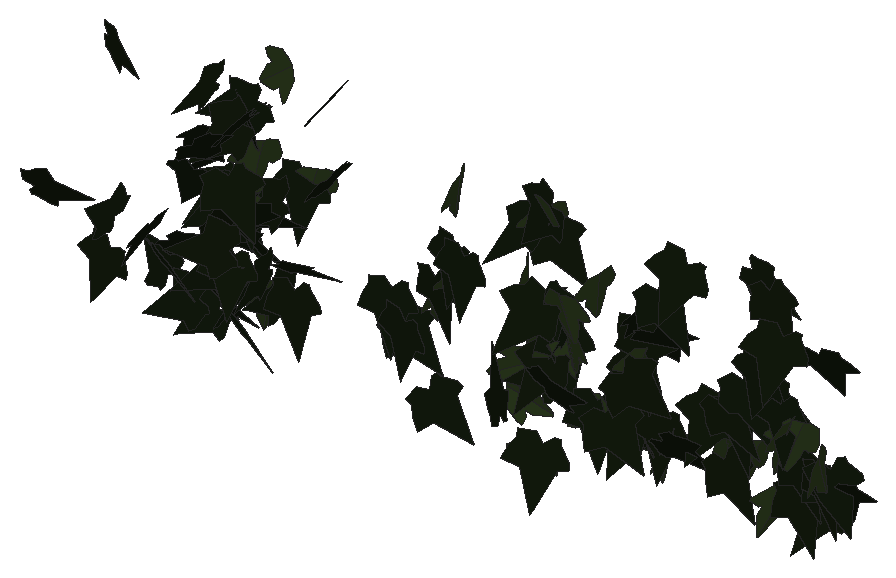
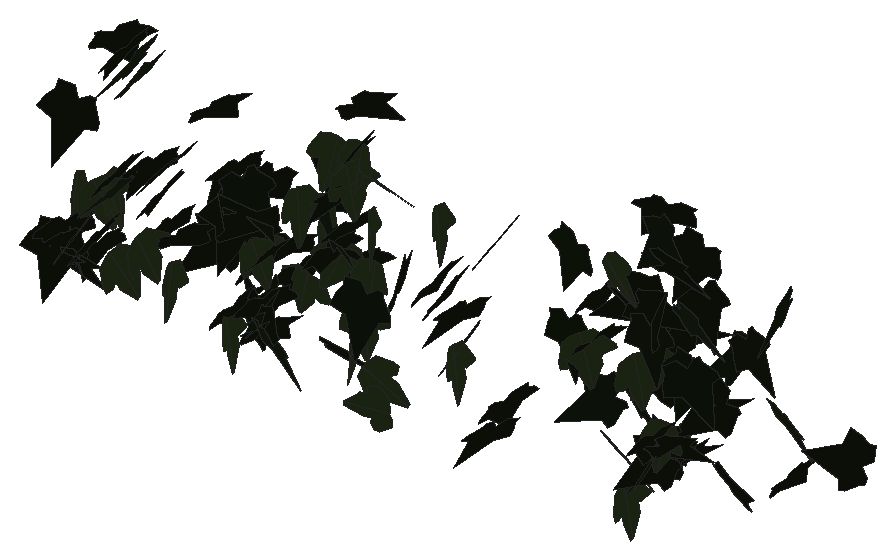
# SketchUp Ruby script. Lengths in inches.
U = 1.inch
M = Sketchup.active_model
def pt(a) = Geom::Point3d.new(a.map { |v| v * U })
def face(e, loops, mat)
  f = e.add_face(loops[0].map { |a| pt(a) })
  loops[1..].each { |l| e.add_face(l.map { |a| pt(a) }).erase! }
  f.material = f.back_material = mat if mat
  f
end
# faces: each face lists its corners as indices into pts; further lists are holes
def faces(e, pts, list, mat = nil) = list.each { |f| face(e, (f[0].is_a?(Array) ? f : [f]).map { |l| l.map { |i| pts[i] } }, mat) }
# xy, xz, yz: faces in a plane at the given z, y or x. An outline is a flat list of corners, or four numbers for a rectangle; further outlines are holes
def ring(l) = l.size == 4 ? [[l[0], l[1]], [l[2], l[1]], [l[2], l[3]], [l[0], l[3]]] : l.each_slice(2).to_a
def flat(e, list, mat, &to3) = list.each { |f| face(e, (f[0].is_a?(Array) ? f : [f]).map { |l| ring(l).map { |u, v| to3.(u, v) } }, mat) }
def xy(e, z, list, mat = nil) = flat(e, list, mat) { |x, y| [x, y, z] }
def xz(e, y, list, mat = nil) = flat(e, list, mat) { |x, z| [x, y, z] }
def yz(e, x, list, mat = nil) = flat(e, list, mat) { |y, z| [x, y, z] }
def lines(e, pts, list) = list.each { |a, b| e.add_line(pt(pts[a]), pt(pts[b])) }
# prism: a flat outline (further loops are holes) pulled along v
def prism(e, loops, v, mat = nil)
  f = face(e, loops, mat); d = Geom::Vector3d.new(v.map { |x| x * U })
  f.pushpull(f.normal.samedirection?(d) ? d.length : -d.length)
end
def box(e, o, s, mat = nil) = prism(e, [[o, [o[0] + s[0], o[1], o[2]], [o[0] + s[0], o[1] + s[1], o[2]], [o[0], o[1] + s[1], o[2]]]], [0, 0, s[2]], mat)
def at(x, y, z, deg = 0) = Geom::Transformation.translation(pt([x, y, z])) * Geom::Transformation.rotation(ORIGIN, Z_AXIS, deg.degrees)
def axes(o, x, y, z) = Geom::Transformation.new([*x, 0, *y, 0, *z, 0, *pt(o).to_a, 1])
def part(name) = M.definitions.add(name)
# library, detail: a bought-in or finely detailed component or shape, given as its bounding box
def library(name, o, s) = part(name).tap { |d| box(d.entities, o, s) }
def detail(e, o, s) = box(e.add_group.entities, o, s)
def put(e, d, t, mat = nil) = e.add_instance(d, t).tap { |i| i.material = mat if mat }
def group(e, t, mat = nil) = e.add_group.tap { |g| g.transformation = t; g.material = mat if mat }.entities
root = M.entities
M.materials.add("efeu1").color = [18, 25, 13]
M.materials.add("efeu2").color = [43, 57, 29]
c1 = part("ivyleaf_9")
p = [[1.54,2.16,1.25],[1.36,2.04,1.19],[-0.21,0.99,0.68],[-0.71,1.11,0.82],[-0.85,0.86,0.67],[-0.8,0.17,0.21],
  [-0.9,-0.01,0.1],[-0.67,-0.16,-0.02],[-0.08,-0.08,-0.05],[-0.03,-0.6,-0.4],[0.65,-0.88,-0.66],[0.83,-0.6,-0.49],
  [1.29,-0.42,-0.43],[1.8125,-0.07,-0.26],[1.21,0.44,0.15]]
faces(c1.entities,p,[[0,1,2,3,4,5,6,7,8,9,10,11,12,13,14]],"efeu1")
c2 = part("ivyleaf_10")
p = [[0,0.5,-0.03],[-0.0625,2.02,-0.43],[-0.19,2.01,-0.46],[-0.54,1.05,-0.29],[-0.52,0.625,-0.18],[-0.83,0.76,-0.28],
  [-1.16,0.64,-0.33],[-1.15,0.33,-0.24],[-0.77,-0.39,0.02],[-0.3,-0.51,0.16],[0.04,-0.48,0.23],[-0.02,2.01,-0.4375],
  [-0.06,2.01,-0.43],[0.04,-0.49,0.23],[0.67,-0.49,0.14],[1.38,0.36,-0.2],[1.375,0.51,-0.24],[0.81,0.65,-0.19],
  [0.62,0.59,-0.15],[0.6,1.09,-0.28],[0.5,1.23,-0.31]]
faces(c2.entities,p,[[0,1,2,3,4,5,6,7,8,9,10],[11,12,0,13,14,15,16,17,18,19,20]],"efeu2")
put(root,c1,axes([1.47,220.37,250.14],[0.26717,-0.08077,0.36252],[0.37184,-0.06164,-0.26897],[0.10521,0.42297,0.03003]))
put(root,c1,axes([2.86,221.11,253.88],[0.33845,-0.15034,-0.27202],[-0.23301,0.15192,-0.35966],[0.22774,0.37887,0.03628]))
put(root,c1,axes([3.35,220.45,249.21],[-0.09676,-0.39725,0.15906],[-0.03153,-0.15019,-0.42349],[0.45865,-0.09413,0.00444]))
put(root,c1,axes([3.79,220.04,250.37],[-0.22269,0.31879,0.22081],[-0.16184,0.15477,-0.39303],[-0.38069,-0.25228,0.03791]))
put(root,c1,axes([4.49,220.96,248.875],[-0.05804,0.18798,0.40413],[-0.27352,0.30338,-0.18905],[-0.37753,-0.24869,0.07484]))
put(root,c1,axes([4.79,222,251.98],[-0.02197,0.39044,-0.19833],[-0.12796,-0.18866,-0.38857],[-0.4515,0.03446,0.11977]))
put(root,c1,axes([5.03,221.85,253.23],[-0.38794,0.2394,-0.05584],[0.00925,-0.08289,-0.44402],[-0.26482,-0.35361,0.06628]))
put(root,c1,axes([5.04,222.57,250.34],[-0.38442,-0.18908,0.17018],[-0.14265,-0.09954,-0.41843],[0.22931,-0.3789,0.025]))
put(root,c1,axes([5.12,221.42,251.63],[0.10444,0.39445,0.16206],[0.00715,0.15841,-0.42128],[-0.45799,0.09242,0.03038]))
put(root,c2,axes([5.23,222.28,250.46],[-0.46353,0.07045,-0.00756],[0.00451,-0.01941,-0.45193],[-0.07636,-0.42882,0.01921]))
put(root,c1,axes([5.52,219.09,251.15],[-0.20155,0.34672,-0.19227],[0.07162,-0.17394,-0.40888],[-0.41828,-0.19686,0.02264]))
put(root,c1,axes([5.3,222.53,250.45],[-0.00279,-0.422,-0.10976],[-0.0063,0.10556,-0.43884],[0.46975,-0.00109,-0.00654]))
put(root,c1,axes([5.28,220.2,250.21],[0.40085,0.17066,0.15545],[0.13196,0.0911,-0.42372],[-0.20644,0.38962,0.03099]))
put(root,c1,axes([5.38,222.49,249.8],[0.27941,-0.33969,-0.08639],[-0.06872,0.05588,-0.44374],[0.37137,0.26592,-0.01711]))
put(root,c1,axes([5.41,222,249.67],[0.44642,0.07487,0.11749],[0.1211,0.01475,-0.43684],[-0.08221,0.42826,-0.00549]))
put(root,c1,axes([5.9,221.89,252.59],[-0.04503,0.43281,-0.01328],[0.00329,-0.01253,-0.4522],[-0.46763,-0.04176,-0.00191]))
put(root,c1,axes([6.08,221.93,253.1],[-0.07388,-0.04884,-0.44387],[-0.27919,-0.34049,0.08362],[-0.37055,0.26628,0.0255]))
put(root,c1,axes([5.97,221.91,252.3],[0.17673,-0.27189,0.30943],[-0.11011,0.28275,0.32704],[-0.42113,-0.18803,0.04434]))
put(root,c2,axes([6,222.24,251.78],[-0.21211,-0.44557,0.08049],[0.00836,-0.09273,-0.49126],[0.4527,-0.20706,0.04679]))
put(root,c1,axes([6.29,221.07,251.24],[-0.48318,0.06047,0.1135],[-0.11269,0.01356,-0.48695],[-0.06197,-0.49614,0.00052]))
put(root,c1,axes([6.19,219.76,252.41],[0.24309,0.17741,-0.34034],[-0.30731,-0.16455,-0.29632],[-0.25919,0.36149,0.03214]))
put(root,c1,axes([5.76,219.03,250.67],[0.36836,-0.2572,0.08541],[0.07301,-0.04674,-0.44425],[0.2823,0.34769,0.00346]))
put(root,c1,axes([6.16,220.58,248.72],[-0.23896,-0.23043,0.30706],[-0.12442,-0.28442,-0.32065],[0.38487,-0.23502,0.08698]))
put(root,c1,axes([6.3,219.71,249.39],[-0.21293,-0.16359,0.36562],[-0.2606,-0.25696,-0.26509],[0.32781,-0.31054,0.02675]))
put(root,c2,axes([6.29,222.2,248.55],[0.00629,-0.49925,0.02656],[0.03614,-0.02604,-0.49801],[0.49865,0.00819,0.03576]))
put(root,c2,axes([6.24,221.17,251.37],[-0.29768,-0.30364,-0.26303],[0.20864,0.16291,-0.42418],[0.3433,-0.3623,0.02972]))
put(root,c1,axes([5.99,220.79,248.86],[0.24443,-0.2247,0.30766],[0.27772,-0.15523,-0.32723],[0.28955,0.33858,0.05415]))
put(root,c2,axes([6.64,222.22,253.96],[0.28525,-0.16574,-0.37572],[-0.32389,0.19042,-0.3299],[0.25245,0.43159,0.00127]))
put(root,c1,axes([6.42,219.5,253.23],[0.25967,0.35435,0.07952],[0.03807,0.06847,-0.44525],[-0.38966,0.24284,0.0095]))
put(root,c1,axes([6.69,220.3,248.96],[-0.0441,0.36683,0.2394],[-0.07348,0.22291,-0.38199],[-0.46192,-0.07048,0.03791]))
put(root,c1,axes([6.78,220.55,253.38],[-0.49533,-0.01361,0.0668],[-0.06663,-0.007,-0.49549],[0.01442,-0.49977,0.00512]))
put(root,c1,axes([6.49,220.02,250.96],[0.10918,0.00626,0.43997],[0.30484,0.32301,-0.07512],[-0.34039,0.29129,0.07384]))
put(root,c1,axes([6.91,220.03,250.25],[-0.06009,-0.06788,-0.4431],[-0.06801,-0.4237,0.07876],[-0.46095,0.07136,0.04615]))
put(root,c1,axes([7.1875,219.61,250.93],[-0.26721,-0.05434,0.36778],[-0.36126,-0.11745,-0.26216],[0.13713,-0.4153,0.02602]))
put(root,c1,axes([6.92,219.92,253.49],[0.17163,0.26338,0.31988],[0.06673,0.31077,-0.30996],[-0.43221,0.15257,0.07916]))
put(root,c1,axes([6.91,220.12,250.38],[-0.13899,-0.40978,-0.07161],[0.02156,0.0659,-0.4467],[0.44825,-0.13023,-0.00072]))
put(root,c1,axes([6.71,220.5,248.67],[0.37999,-0.25111,0.05068],[0.04163,-0.02988,-0.44955],[0.27311,0.35394,-0.002]))
put(root,c1,axes([7.32,221.39,249.08],[-0.3702,0.24263,0.11794],[-0.11124,0.05059,-0.43637],[-0.267,-0.35748,0.01829]))
put(root,c1,axes([7.39,220.69,250.02],[-0.39715,0.19524,-0.13105],[0.12013,-0.05921,-0.433],[-0.22034,-0.38419,0.00014]))
put(root,c2,axes([7.56,222.13,251.7],[-0.31625,-0.36613,0.12622],[-0.04899,-0.12383,-0.48194],[0.38417,-0.3172,0.04245]))
put(root,c1,axes([7.43,221.9375,251.73],[-0.06077,-0.49604,0.01598],[-0.00384,-0.01563,-0.49974],[0.49628,-0.06086,-0.00191]))
put(root,c1,axes([8,220.39,252.03],[-0.43539,0.15483,0.05436],[-0.0519,0.02068,-0.44912],[-0.16869,-0.40599,-0.00215]))
put(root,c1,axes([7.53,221.13,250.01],[0.44332,0.04848,0.14098],[0.12072,0.15081,-0.40811],[-0.09799,0.40513,0.13505]))
put(root,c1,axes([7.5,219.85,251.78],[0.36684,0.06871,0.27344],[0.27106,0.08206,-0.35951],[-0.11254,0.42163,0.02541]))
put(root,c1,axes([8.09,221.88,251.94],[-0.05812,0.43159,0.00808],[-0.00084,0.00773,-0.45233],[-0.46619,-0.05382,-0.00019]))
put(root,c1,axes([8.06,221.7,253.73],[0.04337,0.36601,0.24088],[-0.01546,0.23361,-0.38134],[-0.46754,0.02622,0.03496]))
put(root,c1,axes([8.03,218.65,253.36],[-0.11834,-0.332,-0.35464],[0.26166,0.26397,-0.33444],[0.4093,-0.26475,0.11127]))
put(root,c1,axes([9.52,218.99,250.98],[0.02229,-0.49911,-0.01969],[-0.00044,0.01969,-0.49961],[0.4995,0.02229,0.00044]))
put(root,c1,axes([9.57,222.18,249.65],[-0.02982,-0.49833,-0.02789],[-0.00275,0.0281,-0.4992],[0.4991,-0.02962,-0.00442]))
put(root,c1,axes([9.79,222.29,248.98],[0.14741,-0.36704,-0.30586],[0.02144,0.32485,-0.37949],[0.47729,0.09876,0.11151]))
put(root,c2,axes([10.91,222.18,250.25],[0.08245,-0.48558,-0.08612],[-0.00039,0.08725,-0.49233],[0.49315,0.08125,0.01401]))
put(root,c1,axes([10.87,222.05,250.44],[0.1796,-0.45991,0.07895],[0.01719,-0.07801,-0.49358],[0.46632,0.18,-0.01221]))
put(root,c2,axes([11.66,221.8,253.18],[0.13435,-0.46763,-0.1152],[-0.00065,0.11942,-0.48553],[0.48161,0.13061,0.03148]))
put(root,c1,axes([11.49,221.93,251.4],[0.02545,-0.45539,0.20488],[0.00017,-0.20514,-0.45598],[0.49935,0.02328,-0.01029]))
put(root,c1,axes([11.93,221.66,251.47],[0.02249,-0.48468,0.12075],[0.0066,-0.12058,-0.4852],[0.49945,0.02342,0.00097]))
put(root,c1,axes([12.3,219.2,251.12],[0.03829,-0.45461,0.2046],[0.03718,-0.20202,-0.45586],[0.49714,0.05012,0.01833]))
put(root,c2,axes([13.09,222.22,249.09],[0.25296,0.01557,-0.43101],[-0.4263,0.08479,-0.24713],[0.06539,0.49251,0.05617]))
put(root,c1,axes([12.85,219.42,249.57],[0.17281,-0.34389,-0.31917],[0.00105,0.34042,-0.36622],[0.46919,0.12591,0.11838]))
put(root,c2,axes([12.85,222.25,248.3125],[0.05932,0.01609,0.49621],[0.48469,0.10636,-0.06139],[-0.10753,0.48829,-0.00298]))
put(root,c1,axes([13.43,222.05,250.76],[0.09261,0.48926,0.04529],[0.00191,0.04572,-0.4979],[-0.49135,0.09239,0.0066]))
put(root,c2,axes([13.73,222.05,249.7],[0.16228,-0.415,-0.2268],[0.0164,0.24458,-0.43579],[0.47265,0.134,0.09299]))
put(root,c2,axes([13.8125,221.4,250.93],[-0.47961,0.12763,0.06072],[-0.05992,0.01094,-0.49628],[-0.12801,-0.48331,0.0048]))
put(root,c1,axes([14.19,222.18,249.31],[-0.41889,0.17262,0.2115],[-0.23301,-0.02421,-0.44173],[-0.14226,-0.46863,0.10072]))
put(root,c1,axes([14.05,221.41,253.29],[-0.4968,0.02688,-0.04966],[0.04135,-0.1263,-0.48202],[-0.03846,-0.48304,0.12327]))
put(root,c2,axes([13.9,221.28,252.04],[0.21851,-0.43788,-0.10254],[0.03939,0.1322,-0.48059],[0.448,0.20195,0.09227]))
put(root,c2,axes([14.12,221.46,253.7],[-0.46501,0.17551,0.05444],[-0.04867,0.0252,-0.49699],[-0.17719,-0.46751,-0.00635]))
put(root,c2,axes([14.13,221.77,253.32],[-0.16561,-0.46911,0.05011],[-0.00657,-0.05081,-0.49737],[0.47173,-0.16539,0.01066]))
put(root,c1,axes([14.43,219.74,249.53],[-0.02796,-0.30077,0.39844],[0.04414,0.39601,0.30204],[-0.49726,0.05207,0.00441]))
put(root,c1,axes([14.27,221.68,253.53],[-0.10974,-0.32767,0.36137],[-0.0383,-0.36347,-0.3412],[0.4863,-0.10257,0.05468]))
put(root,c1,axes([14.24,221.77,252.95],[0.13061,-0.40859,-0.2569],[0.05637,0.27723,-0.41227],[0.47934,0.07873,0.11848]))
put(root,c1,axes([14.56,221.15,251.74],[0.11651,-0.45436,-0.17315],[0.02718,0.18386,-0.46417],[0.48548,0.09875,0.06754]))
put(root,c1,axes([15.07,220.71,250.62],[-0.4748,-0.12796,-0.09052],[0.09484,-0.00461,-0.4909],[0.1248,-0.48333,0.02865]))
put(root,c2,axes([15.27,219.84,248.75],[-0.48283,-0.05888,0.11581],[-0.11103,-0.04437,-0.48549],[0.06745,-0.49453,0.02977]))
put(root,c1,axes([15.32,221.02,251.52],[-0.3913,0.24091,-0.1971],[0.17319,-0.09457,-0.45941],[-0.25863,-0.42781,-0.00944]))
put(root,c2,axes([15.09,220.76,250.7],[-0.44054,-0.14074,-0.19004],[0.2038,-0.02211,-0.45605],[0.11996,-0.47927,0.07685]))
put(root,c1,axes([15.04,221.23,251.01],[-0.00964,-0.49252,-0.0856],[-0.00073,0.08563,-0.49261],[0.49991,-0.00937,-0.00237]))
put(root,c2,axes([15.54,221.68,252.2],[-0.06563,-0.49166,-0.06298],[0.01265,0.06184,-0.496],[0.49551,-0.0667,0.00432]))
put(root,c2,axes([15.72,220.52,251.46],[-0.43067,0.22659,0.1148],[-0.1086,0.04003,-0.48642],[-0.22963,-0.44391,0.01474]))
put(root,c1,axes([16.12,221.98,248.87],[-0.30655,0.35645,0.17021],[-0.11909,0.12203,-0.47003],[-0.37662,-0.32871,0.01008]))
put(root,c2,axes([15.97,219.99,252.57],[-0.49646,0.05146,-0.0297],[0.02971,-0.00136,-0.49911],[-0.05145,-0.49734,-0.00171]))
put(root,c1,axes([16.01,219.1875,249.47],[-0.19358,-0.4556,-0.07037],[0.03119,0.0632,-0.49501],[0.45995,-0.19604,0.00395]))
put(root,c1,axes([16.21,218.91,253.06],[-0.35869,-0.31406,0.15069],[-0.10436,-0.10948,-0.47657],[0.33234,-0.37334,0.01298]))
put(root,c2,axes([15.98,220.8,249.71],[0.46097,0.03232,0.19096],[0.18953,0.02611,-0.46195],[-0.03983,0.49827,0.01182]))
put(root,c1,axes([16.29,221.99,248.94],[-0.23568,-0.42741,0.10853],[0.00621,-0.12626,-0.48376],[0.44093,-0.22667,0.06482]))
put(root,c1,axes([16.26,221.9375,249.65],[-0.05766,-0.47716,-0.13783],[0.01969,0.13645,-0.48062],[0.49627,-0.06085,0.00305]))
put(root,c1,axes([16.28,220.74,249.91],[-0.06872,-0.48718,-0.08908],[0.00361,0.08944,-0.49192],[0.49524,-0.06826,-0.00878]))
put(root,c1,axes([16.16,222.02,248.86],[-0.08089,0.08907,0.48531],[0.24888,-0.41728,0.11807],[0.42605,0.26066,0.02317]))
put(root,c1,axes([16.25,221.96,249.39],[0.22258,-0.38534,0.22798],[0.11387,-0.19751,-0.445],[0.43301,0.25001,-0.00017]))
put(root,c2,axes([16.63,221.79,250.7],[-0.07065,-0.47669,0.13331],[-0.00138,-0.13447,-0.48158],[0.49498,-0.06842,0.01768]))
put(root,c1,axes([16.23,219.08,251.01],[0.13173,-0.20881,0.43479],[0.3702,-0.24515,-0.22989],[0.30919,0.38249,0.09002]))
put(root,c1,axes([16.54,221.84,250.38],[-0.05917,-0.4691,0.16261],[0.00371,-0.16417,-0.47227],[0.49647,-0.05468,0.0229]))
put(root,c1,axes([16.69,221.8,251],[-0.25588,-0.06647,0.42439],[0.40702,0.12041,0.26426],[-0.13733,0.48071,-0.00751]))
put(root,c1,axes([17.01,221.66,252.11],[-0.12793,0.42521,-0.22985],[-0.00441,-0.23878,-0.43928],[-0.48334,-0.11037,0.06485]))
put(root,c1,axes([17.04,221.73,251.44],[0.34183,0.35594,-0.08036],[-0.0883,-0.02616,-0.49145],[-0.35406,0.35017,0.04498]))
put(root,c2,axes([17.2,221.94,248.69],[0.13405,-0.47648,-0.07068],[0.00215,0.07396,-0.49449],[0.48169,0.13227,0.02188]))
put(root,c1,axes([17.04,221.98,249.25],[-0.02034,-0.49696,0.05113],[-0.00795,-0.05084,-0.49734],[0.49952,-0.02105,-0.00583]))
put(root,c1,axes([16.97,220.23,250.09],[0.05014,-0.38925,-0.3098],[0.12063,0.31159,-0.37197],[0.48263,-0.03744,0.12516]))
put(root,c1,axes([17.18,221.67,252.49],[0.10876,-0.41748,-0.25276],[0.00875,0.26058,-0.42664],[0.48795,0.08838,0.06399]))
put(root,c1,axes([17.59,220.03,251.36],[0.0837,-0.22339,-0.43942],[-0.03433,0.44199,-0.23123],[0.49175,0.06888,0.05865]))
put(root,c1,axes([18.02,221.52,253.49],[-0.22661,-0.43481,0.09793],[0.00734,-0.11348,-0.4869],[0.44564,-0.21923,0.05782]))
put(root,c1,axes([18.35,220.46,249.83],[0.4793,0.09518,0.10587],[0.10305,0.0246,-0.48865],[-0.09822,0.49024,0.00397]))
put(root,c2,axes([18.71,221.97,249.42],[0.09605,-0.46274,-0.16323],[0.05481,0.17541,-0.465],[0.48762,0.07143,0.08442]))
put(root,c1,axes([18.76,221.68,250.23],[-0.28263,-0.40112,0.09603],[0.00076,-0.11692,-0.48614],[0.41245,-0.27465,0.0667]))
put(root,c2,axes([19.75,221.7,249.58],[-0.04856,-0.4521,0.20796],[0.02701,-0.21103,-0.45248],[0.4969,-0.03272,0.04492]))
put(root,c1,axes([19.63,221.18,250.73],[0.14188,-0.4794,-0.00659],[-0.00309,0.00596,-0.49995],[0.47944,0.14191,-0.00128]))
put(root,c1,axes([19.77,220.68,249.75],[0.15758,-0.41207,-0.2353],[-0.04529,0.23375,-0.43967],[0.47235,0.15988,0.03634]))
put(root,c1,axes([19.75,220.58,251.21],[0.24891,-0.39622,-0.17623],[0.00289,0.20471,-0.45616],[0.43363,0.22607,0.1042]))
put(root,c1,axes([19.82,221.24,251.44],[0.07857,-0.43604,-0.23173],[0.01346,0.23645,-0.44035],[0.49361,0.06295,0.04889]))
put(root,c1,axes([19.9375,221.46,254.06],[0.37242,-0.26478,-0.20297],[-0.07752,0.22719,-0.43861],[0.32449,0.35816,0.12817]))
put(root,c1,axes([20.08,221.74,251.14],[0.37494,-0.26587,-0.19681],[-0.04233,0.25648,-0.42711],[0.32807,0.33695,0.16982]))
put(root,c2,axes([20.58,221.52,248.84],[-0.10613,-0.42724,0.23707],[-0.05049,-0.23171,-0.44018],[0.48599,-0.11737,0.00604]))
put(root,c1,axes([20.57,221.625,251.01],[0.03596,-0.49205,0.08121],[0.0101,-0.08068,-0.49334],[0.4986,0.03712,0.00413]))
put(root,c1,axes([20.58,221.2,253.89],[0.15395,-0.46314,-0.10863],[-0.00798,0.11165,-0.48731],[0.47564,0.15177,0.02698]))
put(root,c2,axes([20.82,221.4,250.56],[0.11277,-0.48101,0.07687],[0.0264,-0.07275,-0.49397],[0.4864,0.11547,0.00899]))
put(root,c2,axes([20.99,221.63,250.48],[-0.27918,-0.3639,0.19909],[-0.02564,-0.22438,-0.44609],[0.41401,-0.25929,0.10662]))
put(root,c1,axes([20.74,221.86,249.68],[0.18593,-0.44788,-0.12181],[-0.02513,0.12132,-0.48441],[0.46346,0.18625,0.02261]))
put(root,c1,axes([21.05,221.55,249.14],[0.04613,-0.47078,-0.162],[-0.01991,0.16082,-0.47301],[0.49747,0.05009,-0.00391]))
put(root,c1,axes([21.03,220.33,252.53],[-0.04387,-0.41528,0.27499],[0.08239,-0.27831,-0.40713],[0.49121,0.00959,0.09285]))
put(root,c1,axes([21.61,221.99,248.91],[-0.47965,-0.12961,-0.05601],[0.06346,-0.0207,-0.49552],[0.12613,-0.48246,0.03631]))
put(root,c1,axes([21.32,221.96,249.45],[0.17967,-0.4649,0.03983],[-0.00075,-0.04297,-0.49815],[0.4666,0.17894,-0.01614]))
put(root,c1,axes([21.51,221.7,252.48],[0.42014,0.22557,-0.15034],[-0.13394,-0.06835,-0.47685],[-0.23568,0.44096,0.00299]))
put(root,c1,axes([21.57,220.3125,253.51],[-0.25336,-0.42735,-0.05646],[0.02057,0.05342,-0.49671],[0.43057,-0.25401,-0.00949]))
put(root,c1,axes([21.73,221.91,249.25],[0.36042,0.31164,-0.15158],[-0.14586,-0.06196,-0.47422],[-0.31435,0.38606,0.04625]))
put(root,c1,axes([21.625,221.91,249.625],[-0.01498,-0.43267,-0.25015],[0.02938,0.24906,-0.43256],[0.49891,-0.02766,0.01796]))
put(root,c2,axes([21.84,221.23,250.19],[0.14771,-0.42771,-0.21271],[0.03777,0.23241,-0.44109],[0.47619,0.11424,0.10097]))
